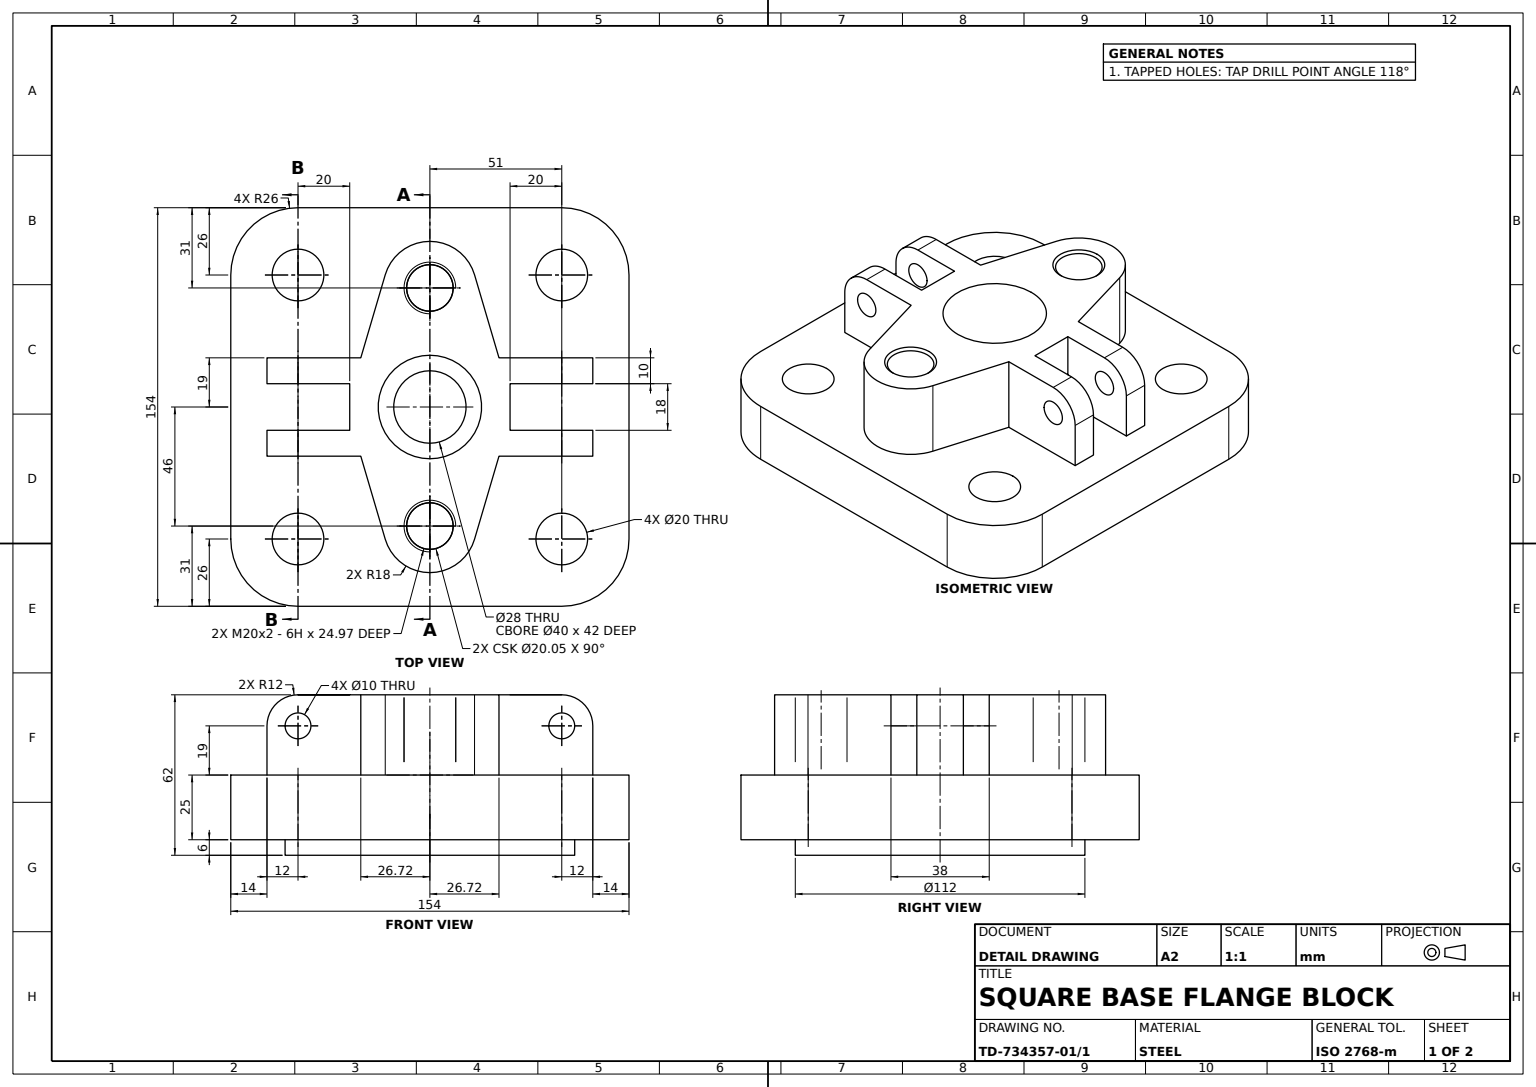
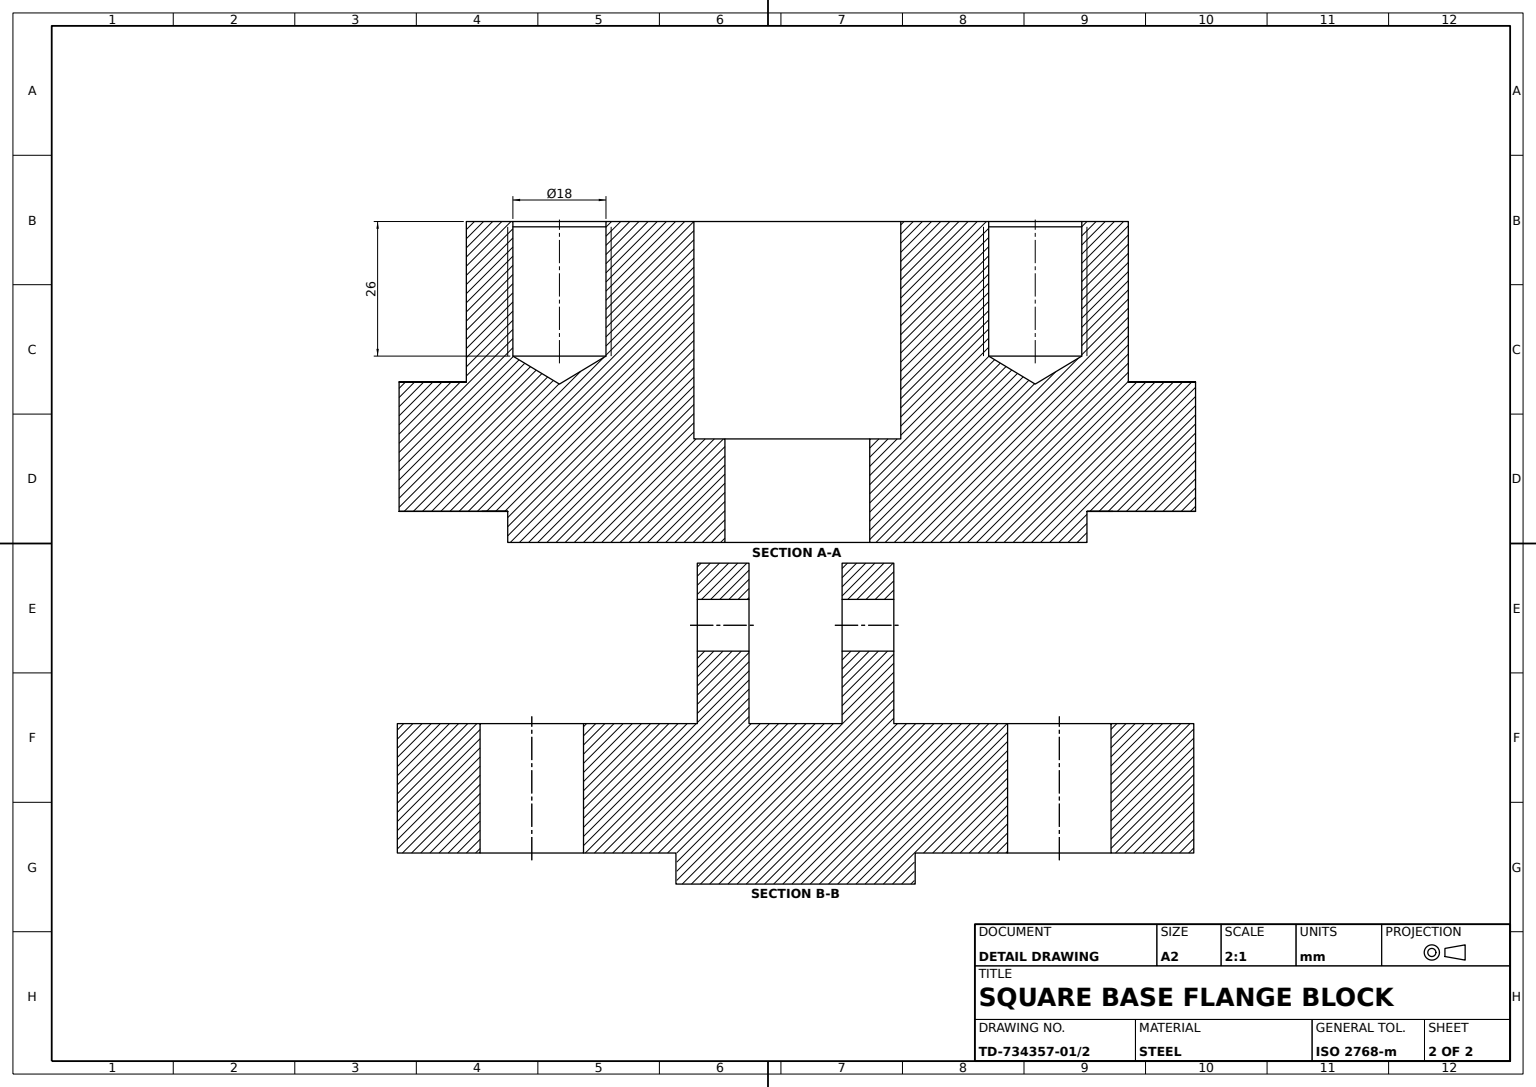
solid
v1 (0,54.975,-37)
v2 (0,56,-35.975)
e1 v1 v2 LINE
v3 (0,54.975,-55)
e2 v3 v1 CIRCLE(AX(P(0,54.975,-46),D(0,1,0),D(0,0,1)),9)
v4 (0,56,-56.025)
e3 v3 v4 LINE
e4 v4 v2 CIRCLE(AX(P(0,56,-46),D(0,1,0),D(0,0,1)),10.025)
face CONE(AX(P(0,56,-46),D(0,1,0),D(0,0,1)),10.025,0.785398163) rev [-e1 -e2 e3 e4]
v5 (51,25,-77)
v6 (51,0,-77)
e5 v5 v6 LINE
v7 (77,25,-51)
e6 v7 v5 CIRCLE(AX(P(51,25,-51),D(0,1,0),D(0,0,-1)),26)
v8 (77,0,-51)
e7 v7 v8 LINE
e8 v8 v6 CIRCLE(AX(P(51,0,-51),D(0,1,0),D(0,0,-1)),26)
face CYL(AX(P(51,25,-51),D(0,-1,0),D(0,0,-1)),26) [-e5 -e6 e7 e8]
v9 (-51,0,-61)
v10 (-51,0,-41)
e9 v9 v10 CIRCLE(AX(P(-51,0,-51),D(0,-1,0),D(0,0,-1)),10)
v11 (-51,25,-41)
e10 v10 v11 LINE
v12 (-51,25,-61)
e11 v11 v12 CIRCLE(AX(P(-51,25,-51),D(0,1,0),D(0,0,1)),10)
e12 v9 v12 LINE
face CYL(AX(P(-51,-17,-51),D(0,1,0),D(0,0,1)),10) rev [e9 e10 e11 -e12]
e13 v12 v11 CIRCLE(AX(P(-51,25,-51),D(0,1,0),D(0,0,1)),10)
v13 (63,25,9)
v14 (31,25,9)
e14 v13 v14 LINE
v15 (63,25,19)
e15 v15 v13 LINE
v16 (26.719654,25,19)
e16 v16 v15 LINE
v17 (17.266235,25,51.086957)
e17 v17 v16 LINE
v18 (-17.266235,25,51.086957)
e18 v18 v17 CIRCLE(AX(P(0,25,46),D(0,1,0),D(0,0,1)),18)
v19 (-26.719654,25,19)
e19 v19 v18 LINE
v20 (-63,25,19)
e20 v20 v19 LINE
v21 (-63,25,9)
e21 v21 v20 LINE
v22 (-31,25,9)
e22 v22 v21 LINE
v23 (-31,25,-9)
e23 v23 v22 LINE
v24 (-63,25,-9)
e24 v24 v23 LINE
v25 (-63,25,-19)
e25 v25 v24 LINE
v26 (-26.719654,25,-19)
e26 v26 v25 LINE
v27 (-17.266235,25,-51.086957)
e27 v27 v26 LINE
v28 (0,25,-64)
e28 v28 v27 CIRCLE(AX(P(0,25,-46),D(0,1,0),D(0,0,1)),18)
v29 (17.266235,25,-51.086957)
e29 v29 v28 CIRCLE(AX(P(0,25,-46),D(0,1,0),D(0,0,1)),18)
v30 (26.719654,25,-19)
e30 v30 v29 LINE
v31 (63,25,-19)
e31 v31 v30 LINE
v32 (63,25,-9)
e32 v32 v31 LINE
v33 (31,25,-9)
e33 v33 v32 LINE
e34 v14 v33 LINE
v34 (-77,25,-51)
v35 (-77,25,51)
e35 v34 v35 LINE
v36 (-51,25,77)
e36 v35 v36 CIRCLE(AX(P(-51,25,51),D(0,1,0),D(0,0,-1)),26)
v37 (51,25,77)
e37 v36 v37 LINE
v38 (77,25,51)
e38 v37 v38 CIRCLE(AX(P(51,25,51),D(0,1,0),D(0,0,1)),26)
e39 v38 v7 LINE
v39 (-51,25,-77)
e40 v5 v39 LINE
e41 v39 v34 CIRCLE(AX(P(-51,25,-51),D(0,1,0),D(0,0,-1)),26)
v40 (51,25,-61)
v41 (51,25,-41)
e42 v40 v41 CIRCLE(AX(P(51,25,-51),D(0,1,0),D(0,0,1)),10)
e43 v41 v40 CIRCLE(AX(P(51,25,-51),D(0,1,0),D(0,0,1)),10)
v42 (51,25,41)
v43 (51,25,61)
e44 v42 v43 CIRCLE(AX(P(51,25,51),D(0,1,0),D(0,0,1)),10)
e45 v43 v42 CIRCLE(AX(P(51,25,51),D(0,1,0),D(0,0,1)),10)
v44 (-51,25,41)
v45 (-51,25,61)
e46 v44 v45 CIRCLE(AX(P(-51,25,51),D(0,1,0),D(0,0,1)),10)
e47 v45 v44 CIRCLE(AX(P(-51,25,51),D(0,1,0),D(0,0,1)),10)
face PLANE(AX(P(-51,25,51),D(0,-1,0),D(0,0,-1))) rev [-e13 -e11] [-e14 -e15 -e16 -e17 -e18 -e19 -e20 -e21 -e22 -e23 -e24 -e25 -e26 -e27 -e28 -e29 -e30 -e31 -e32 -e33 -e34] [e35 e36 e37 e38 e39 e6 e40 e41] [-e42 -e43] [-e44 -e45] [-e46 -e47]
v46 (0,30,-55)
e48 v46 v3 LINE
v47 (0,30,-37)
e49 v47 v1 LINE
e50 v46 v47 CIRCLE(AX(P(0,30,-46),D(0,1,0),D(0,0,1)),9)
face CYL(AX(P(0,56,-46),D(0,1,0),D(0,0,1)),9) rev [e48 e2 -e49 -e50]
v48 (-63,44,-9)
v49 (-63,44,-19)
e51 v48 v49 LINE
v50 (-51,56,-9)
e52 v50 v48 CIRCLE(AX(P(-51,44,-9),D(0,0,1),D(-1,0,0)),12)
v51 (-51,56,-19)
e53 v51 v50 LINE
e54 v49 v51 CIRCLE(AX(P(-51,44,-19),D(0,0,-1),D(1,0,0)),12)
face CYL(AX(P(-51,44,-46),D(0,0,-1),D(-1,0,0)),12) [-e51 -e52 -e53 -e54]
v52 (-51,56,19)
v53 (-26.719654,56,19)
e55 v52 v53 LINE
v54 (-63,44,19)
e56 v52 v54 CIRCLE(AX(P(-51,44,19),D(0,0,1),D(-1,0,0)),12)
e57 v54 v20 LINE
e58 v53 v19 LINE
v55 (-56,44,19)
v56 (-46,44,19)
e59 v55 v56 CIRCLE(AX(P(-51,44,19),D(0,0,1),D(1,0,0)),5)
e60 v56 v55 CIRCLE(AX(P(-51,44,19),D(0,0,1),D(1,0,0)),5)
face PLANE(AX(P(-63,56,19),D(0,0,-1),D(-1,0,0))) rev [-e55 e56 e57 e20 -e58] [-e59 -e60]
e61 v48 v24 LINE
e62 v49 v25 LINE
face PLANE(AX(P(-63,56,-9),D(1,0,0),D(0,0,-1))) rev [-e61 e51 e62 e25]
v57 (-46,44,-19)
v58 (-46,44,-9)
e63 v57 v58 LINE
v59 (-56,44,-19)
e64 v59 v57 CIRCLE(AX(P(-51,44,-19),D(0,0,1),D(1,0,0)),5)
v60 (-56,44,-9)
e65 v59 v60 LINE
e66 v58 v60 CIRCLE(AX(P(-51,44,-9),D(0,0,-1),D(-1,0,0)),5)
face CYL(AX(P(-51,44,-77),D(0,0,1),D(1,0,0)),5) rev [-e63 -e64 e65 -e66]
v61 (0,0,-56)
v62 (0,0,56)
e67 v61 v62 CIRCLE(AX(P(0,0,0),D(0,-1,0),D(0,0,-1)),56)
v63 (0,-6,56)
e68 v63 v62 LINE
v64 (0,-6,-56)
e69 v64 v63 CIRCLE(AX(P(0,-6,0),D(0,-1,0),D(0,0,-1)),56)
e70 v64 v61 LINE
face CYL(AX(P(0,-6,0),D(0,1,0),D(0,0,1)),56) [e67 -e68 -e69 e70]
v65 (0,-6,-14)
v66 (0,14,-14)
e71 v65 v66 LINE
v67 (0,14,14)
e72 v66 v67 CIRCLE(AX(P(0,14,0),D(0,1,0),D(0,0,1)),14)
v68 (0,-6,14)
e73 v68 v67 LINE
e74 v68 v65 CIRCLE(AX(P(0,-6,0),D(0,-1,0),D(0,0,-1)),14)
face CYL(AX(P(0,-28,0),D(0,1,0),D(0,0,1)),14) rev [e71 e72 -e73 e74]
v69 (0,56,56.025)
v70 (0,56,35.975)
e75 v69 v70 CIRCLE(AX(P(0,56,46),D(0,1,0),D(0,0,1)),10.025)
v71 (0,54.975,37)
e76 v71 v70 LINE
v72 (0,54.975,55)
e77 v72 v71 CIRCLE(AX(P(0,54.975,46),D(0,1,0),D(0,0,1)),9)
e78 v72 v69 LINE
face CONE(AX(P(0,56,46),D(0,1,0),D(0,0,1)),10.025,0.785398163) rev [e75 -e76 -e77 e78]
e79 v62 v61 CIRCLE(AX(P(0,0,0),D(0,-1,0),D(0,0,-1)),56)
e80 v63 v64 CIRCLE(AX(P(0,-6,0),D(0,-1,0),D(0,0,-1)),56)
face CYL(AX(P(0,-6,0),D(0,1,0),D(0,0,1)),56) [e79 -e70 -e80 e68]
e81 v70 v69 CIRCLE(AX(P(0,56,46),D(0,1,0),D(0,0,1)),10.025)
v73 (0,56,-20)
v74 (0,56,20)
e82 v73 v74 CIRCLE(AX(P(0,56,0),D(0,1,0),D(0,0,1)),20)
e83 v74 v73 CIRCLE(AX(P(0,56,0),D(0,1,0),D(0,0,1)),20)
e84 v2 v4 CIRCLE(AX(P(0,56,-46),D(0,1,0),D(0,0,1)),10.025)
v75 (-51,56,9)
e85 v75 v52 LINE
v76 (-17.266235,56,51.086957)
e86 v53 v76 LINE
v77 (17.266235,56,51.086957)
e87 v76 v77 CIRCLE(AX(P(0,56,46),D(0,1,0),D(0,0,1)),18)
v78 (26.719654,56,19)
e88 v77 v78 LINE
v79 (51,56,19)
e89 v78 v79 LINE
v80 (51,56,9)
e90 v79 v80 LINE
v81 (31,56,9)
e91 v80 v81 LINE
v82 (31,56,-9)
e92 v81 v82 LINE
v83 (51,56,-9)
e93 v82 v83 LINE
v84 (51,56,-19)
e94 v83 v84 LINE
v85 (26.719654,56,-19)
e95 v84 v85 LINE
v86 (17.266235,56,-51.086957)
e96 v85 v86 LINE
v87 (0,56,-64)
e97 v86 v87 CIRCLE(AX(P(0,56,-46),D(0,1,0),D(0,0,1)),18)
v88 (-17.266235,56,-51.086957)
e98 v87 v88 CIRCLE(AX(P(0,56,-46),D(0,1,0),D(0,0,1)),18)
v89 (-26.719654,56,-19)
e99 v88 v89 LINE
e100 v89 v51 LINE
v90 (-31,56,-9)
e101 v50 v90 LINE
v91 (-31,56,9)
e102 v90 v91 LINE
e103 v91 v75 LINE
face PLANE(AX(P(0,56,-46),D(0,1,0),D(0,0,1))) [-e81 -e75] [-e82 -e83] [-e84 -e4] [e85 e55 e86 e87 e88 e89 e90 e91 e92 e93 e94 e95 e96 e97 e98 e99 e100 e53 e101 e102 e103]
v92 (46,44,-19)
v93 (56,44,-19)
e104 v92 v93 CIRCLE(AX(P(51,44,-19),D(0,0,1),D(1,0,0)),5)
v94 (46,44,-9)
e105 v92 v94 LINE
v95 (56,44,-9)
e106 v95 v94 CIRCLE(AX(P(51,44,-9),D(0,0,-1),D(-1,0,0)),5)
e107 v93 v95 LINE
face CYL(AX(P(51,44,-77),D(0,0,1),D(1,0,0)),5) rev [-e104 e105 -e106 -e107]
v96 (63,44,-9)
e108 v96 v32 LINE
e109 v96 v83 CIRCLE(AX(P(51,44,-9),D(0,0,1),D(-1,0,0)),12)
e110 v82 v33 LINE
e111 v94 v95 CIRCLE(AX(P(51,44,-9),D(0,0,-1),D(-1,0,0)),5)
face PLANE(AX(P(31,56,-9),D(0,0,-1),D(-1,0,0))) rev [-e108 e109 -e93 e110 e33] [e106 e111]
v97 (-56,44,9)
e112 v97 v55 LINE
v98 (-46,44,9)
e113 v98 v56 LINE
e114 v97 v98 CIRCLE(AX(P(-51,44,9),D(0,0,1),D(1,0,0)),5)
face CYL(AX(P(-51,44,-77),D(0,0,1),D(1,0,0)),5) rev [e112 e59 -e113 -e114]
e115 v65 v68 CIRCLE(AX(P(0,-6,0),D(0,-1,0),D(0,0,-1)),14)
face PLANE(AX(P(0,-6,0),D(0,-1,0),D(0,0,-1))) [-e74 -e115] [e80 e69]
v99 (51,0,61)
e116 v99 v43 LINE
v100 (51,0,41)
e117 v99 v100 CIRCLE(AX(P(51,0,51),D(0,-1,0),D(0,0,-1)),10)
e118 v100 v42 LINE
face CYL(AX(P(51,-17,51),D(0,1,0),D(0,0,1)),10) rev [-e116 e117 e118 e44]
e119 v1 v3 CIRCLE(AX(P(0,54.975,-46),D(0,1,0),D(0,0,1)),9)
face CONE(AX(P(0,56,-46),D(0,1,0),D(0,0,1)),10.025,0.785398163) rev [e1 e84 -e3 -e119]
v101 (-51,0,77)
v102 (51,0,77)
e120 v101 v102 LINE
e121 v37 v102 LINE
e122 v36 v101 LINE
face PLANE(AX(P(-51,25,77),D(0,0,-1),D(-1,0,0))) rev [e120 -e121 -e37 e122]
v103 (-63,44,9)
e123 v54 v103 LINE
e124 v103 v21 LINE
face PLANE(AX(P(-63,56,9),D(1,0,0),D(0,0,-1))) rev [-e57 e123 e124 e21]
v104 (46,44,9)
v105 (46,44,19)
e125 v104 v105 LINE
v106 (56,44,9)
e126 v106 v104 CIRCLE(AX(P(51,44,9),D(0,0,1),D(1,0,0)),5)
v107 (56,44,19)
e127 v106 v107 LINE
e128 v107 v105 CIRCLE(AX(P(51,44,19),D(0,0,1),D(1,0,0)),5)
face CYL(AX(P(51,44,-77),D(0,0,1),D(1,0,0)),5) rev [-e125 -e126 e127 e128]
e129 v98 v97 CIRCLE(AX(P(-51,44,9),D(0,0,1),D(1,0,0)),5)
face CYL(AX(P(-51,44,-77),D(0,0,1),D(1,0,0)),5) rev [-e112 -e129 e113 e60]
v108 (51,0,-61)
e130 v108 v40 LINE
v109 (51,0,-41)
e131 v108 v109 CIRCLE(AX(P(51,0,-51),D(0,-1,0),D(0,0,-1)),10)
e132 v109 v41 LINE
face CYL(AX(P(51,-17,-51),D(0,1,0),D(0,0,1)),10) rev [e43 -e130 e131 e132]
v110 (0,14,-20)
v111 (0,14,20)
e133 v110 v111 CIRCLE(AX(P(0,14,0),D(0,1,0),D(0,0,1)),20)
e134 v111 v110 CIRCLE(AX(P(0,14,0),D(0,1,0),D(0,0,1)),20)
e135 v67 v66 CIRCLE(AX(P(0,14,0),D(0,1,0),D(0,0,1)),14)
face PLANE(AX(P(0,14,0),D(0,1,0),D(0,0,1))) [e133 e134] [-e72 -e135]
e136 v111 v74 LINE
e137 v110 v73 LINE
face CYL(AX(P(0,14,0),D(0,1,0),D(0,0,1)),20) rev [e136 e83 -e137 -e134]
v112 (63,44,-19)
e138 v112 v96 LINE
e139 v84 v112 CIRCLE(AX(P(51,44,-19),D(0,0,-1),D(1,0,0)),12)
face CYL(AX(P(51,44,-46),D(0,0,1),D(1,0,0)),12) [-e109 -e138 -e139 -e94]
e140 v77 v17 LINE
e141 v78 v16 LINE
face PLANE(AX(P(17.266235,56,51.086957),D(-0.959235281,0,-0.282608696),D(-0.282608696,0,0.959235281))) rev [e140 e17 -e141 -e88]
e142 v71 v72 CIRCLE(AX(P(0,54.975,46),D(0,1,0),D(0,0,1)),9)
face CONE(AX(P(0,56,46),D(0,1,0),D(0,0,1)),10.025,0.785398163) rev [e81 -e78 -e142 e76]
v113 (-51,0,41)
e143 v113 v44 LINE
v114 (-51,0,61)
e144 v113 v114 CIRCLE(AX(P(-51,0,51),D(0,-1,0),D(0,0,-1)),10)
e145 v114 v45 LINE
face CYL(AX(P(-51,-17,51),D(0,1,0),D(0,0,1)),10) rev [-e143 e144 e145 e47]
v115 (0,24.592254,-46)
e146 v115 v47 LINE
e147 v47 v46 CIRCLE(AX(P(0,30,-46),D(0,1,0),D(0,0,1)),9)
e148 v115 v46 LINE
face CONE(AX(P(0,30,-46),D(0,1,0),D(0,0,1)),9,1.029744259) rev [e146 e147 -e148]
e149 v104 v106 CIRCLE(AX(P(51,44,9),D(0,0,1),D(1,0,0)),5)
e150 v81 v14 LINE
v116 (63,44,9)
e151 v80 v116 CIRCLE(AX(P(51,44,9),D(0,0,-1),D(1,0,0)),12)
e152 v116 v13 LINE
face PLANE(AX(P(31,56,9),D(0,0,1),D(1,0,0))) rev [e149 e126] [-e150 -e91 e151 e152 e14]
e153 v87 v28 LINE
e154 v86 v29 LINE
face CYL(AX(P(0,56,-46),D(0,-1,0),D(0,0,-1)),18) [e29 -e153 -e97 e154]
e155 v105 v107 CIRCLE(AX(P(51,44,19),D(0,0,1),D(1,0,0)),5)
face CYL(AX(P(51,44,-77),D(0,0,1),D(1,0,0)),5) rev [e125 e155 -e127 -e149]
e156 v10 v9 CIRCLE(AX(P(-51,0,-51),D(0,-1,0),D(0,0,-1)),10)
face CYL(AX(P(-51,-17,-51),D(0,1,0),D(0,0,1)),10) rev [e12 e13 -e10 e156]
v117 (-77,0,51)
e157 v35 v117 LINE
e158 v117 v101 CIRCLE(AX(P(-51,0,51),D(0,1,0),D(0,0,-1)),26)
face CYL(AX(P(-51,25,51),D(0,-1,0),D(0,0,-1)),26) [-e36 e157 e158 -e122]
e159 v93 v92 CIRCLE(AX(P(51,44,-19),D(0,0,1),D(1,0,0)),5)
e160 v85 v30 LINE
e161 v112 v31 LINE
face PLANE(AX(P(63,56,-19),D(0,0,1),D(1,0,0))) rev [e159 e104] [e31 -e160 -e95 e139 e161]
face PLANE(AX(P(63,56,-9),D(-1,0,0),D(0,0,1))) rev [-e161 e138 e108 e32]
v118 (63,44,19)
e162 v116 v118 LINE
e163 v118 v79 CIRCLE(AX(P(51,44,19),D(0,0,1),D(-1,0,0)),12)
face CYL(AX(P(51,44,-46),D(0,0,1),D(1,0,0)),12) [-e162 -e151 -e90 -e163]
e164 v76 v18 LINE
face PLANE(AX(P(-17.266235,56,51.086957),D(0.959235281,0,-0.282608696),D(-0.282608696,0,-0.959235281))) rev [e19 -e164 -e86 e58]
e165 v57 v59 CIRCLE(AX(P(-51,44,-19),D(0,0,1),D(1,0,0)),5)
e166 v89 v26 LINE
face PLANE(AX(P(-63,56,-19),D(0,0,1),D(1,0,0))) rev [e165 e64] [e166 e26 -e62 e54 -e100]
face PLANE(AX(P(17.266235,56,-51.086957),D(-0.959235281,0,0.282608696),D(0.282608696,0,0.959235281))) rev [-e154 -e96 e160 e30]
e167 v118 v15 LINE
face PLANE(AX(P(63,56,19),D(0,0,-1),D(-1,0,0))) rev [-e128 -e155] [e16 -e167 e163 -e89 e141]
face CYL(AX(P(0,56,46),D(0,-1,0),D(0,0,-1)),18) [e18 -e140 -e87 e164]
v119 (0,30,55)
v120 (0,30,37)
e168 v119 v120 CIRCLE(AX(P(0,30,46),D(0,1,0),D(0,0,1)),9)
e169 v119 v72 LINE
e170 v120 v71 LINE
face CYL(AX(P(0,56,46),D(0,1,0),D(0,0,1)),9) rev [-e168 e169 e77 -e170]
face PLANE(AX(P(31,56,9),D(-1,0,0),D(0,0,1))) rev [-e110 -e92 e150 e34]
e171 v103 v75 CIRCLE(AX(P(-51,44,9),D(0,0,-1),D(1,0,0)),12)
e172 v91 v22 LINE
face PLANE(AX(P(-31,56,9),D(0,0,1),D(1,0,0))) rev [-e124 e171 -e103 e172 e22] [e129 e114]
e173 v100 v99 CIRCLE(AX(P(51,0,51),D(0,-1,0),D(0,0,-1)),10)
face CYL(AX(P(51,-17,51),D(0,1,0),D(0,0,1)),10) rev [-e118 e173 e116 e45]
e174 v88 v27 LINE
face CYL(AX(P(0,56,-46),D(0,-1,0),D(0,0,-1)),18) [-e174 -e98 e153 e28]
face CONE(AX(P(0,30,-46),D(0,1,0),D(0,0,1)),9,1.029744259) rev [-e146 e148 e50]
face CYL(AX(P(0,56,-46),D(0,1,0),D(0,0,1)),9) rev [e49 e119 -e48 -e147]
face CYL(AX(P(0,-28,0),D(0,1,0),D(0,0,1)),14) rev [e135 -e71 e115 e73]
e175 v90 v23 LINE
face PLANE(AX(P(-31,56,9),D(1,0,0),D(0,0,-1))) rev [-e102 e175 e23 -e172]
face PLANE(AX(P(-17.266235,56,-51.086957),D(0.959235281,0,0.282608696),D(0.282608696,0,-0.959235281))) rev [e27 -e166 -e99 e174]
e176 v60 v58 CIRCLE(AX(P(-51,44,-9),D(0,0,-1),D(-1,0,0)),5)
face PLANE(AX(P(-31,56,-9),D(0,0,-1),D(-1,0,0))) rev [e66 e176] [e61 e24 -e175 -e101 e52]
v121 (77,0,51)
e177 v38 v121 LINE
e178 v121 v8 LINE
face PLANE(AX(P(77,25,51),D(-1,0,0),D(0,0,1))) rev [-e7 -e39 e177 e178]
face CYL(AX(P(0,14,0),D(0,1,0),D(0,0,1)),20) rev [-e136 -e133 e137 e82]
v122 (0,24.592254,46)
e179 v122 v120 LINE
e180 v122 v119 LINE
face CONE(AX(P(0,30,46),D(0,1,0),D(0,0,1)),9,1.029744259) rev [e168 -e179 e180]
face CYL(AX(P(-51,44,-77),D(0,0,1),D(1,0,0)),5) rev [e63 -e176 -e65 -e165]
face CYL(AX(P(-51,44,-46),D(0,0,-1),D(-1,0,0)),12) [-e171 -e123 -e56 -e85]
e181 v102 v121 CIRCLE(AX(P(51,0,51),D(0,1,0),D(0,0,1)),26)
face CYL(AX(P(51,25,51),D(0,-1,0),D(0,0,-1)),26) [e121 e181 -e177 -e38]
e182 v120 v119 CIRCLE(AX(P(0,30,46),D(0,1,0),D(0,0,1)),9)
face CYL(AX(P(0,56,46),D(0,1,0),D(0,0,1)),9) rev [e142 -e169 -e182 e170]
e183 v114 v113 CIRCLE(AX(P(-51,0,51),D(0,-1,0),D(0,0,-1)),10)
face CYL(AX(P(-51,-17,51),D(0,1,0),D(0,0,1)),10) rev [-e145 e183 e143 e46]
face CYL(AX(P(51,44,-77),D(0,0,1),D(1,0,0)),5) rev [-e159 e107 -e111 -e105]
v123 (-51,0,-77)
e184 v6 v123 LINE
e185 v39 v123 LINE
face PLANE(AX(P(-51,25,-77),D(0,0,1),D(1,0,0))) rev [e184 -e185 -e40 e5]
v124 (-77,0,-51)
e186 v124 v117 LINE
e187 v34 v124 LINE
face PLANE(AX(P(-77,25,51),D(1,0,0),D(0,0,-1))) rev [e186 -e157 -e35 e187]
e188 v109 v108 CIRCLE(AX(P(51,0,-51),D(0,-1,0),D(0,0,-1)),10)
face CYL(AX(P(51,-17,-51),D(0,1,0),D(0,0,1)),10) rev [e130 e42 -e132 e188]
e189 v123 v124 CIRCLE(AX(P(-51,0,-51),D(0,1,0),D(0,0,-1)),26)
face PLANE(AX(P(-51,0,51),D(0,-1,0),D(0,0,-1))) [-e188 -e131] [-e8 -e178 -e181 -e120 -e158 -e186 -e189 -e184] [-e67 -e79] [-e173 -e117] [-e183 -e144] [-e9 -e156]
face CONE(AX(P(0,30,46),D(0,1,0),D(0,0,1)),9,1.029744259) rev [-e180 e179 e182]
face PLANE(AX(P(63,56,9),D(-1,0,0),D(0,0,1))) rev [e15 -e152 e162 e167]
face CYL(AX(P(-51,25,-51),D(0,-1,0),D(0,0,-1)),26) [-e187 -e41 e185 e189]
